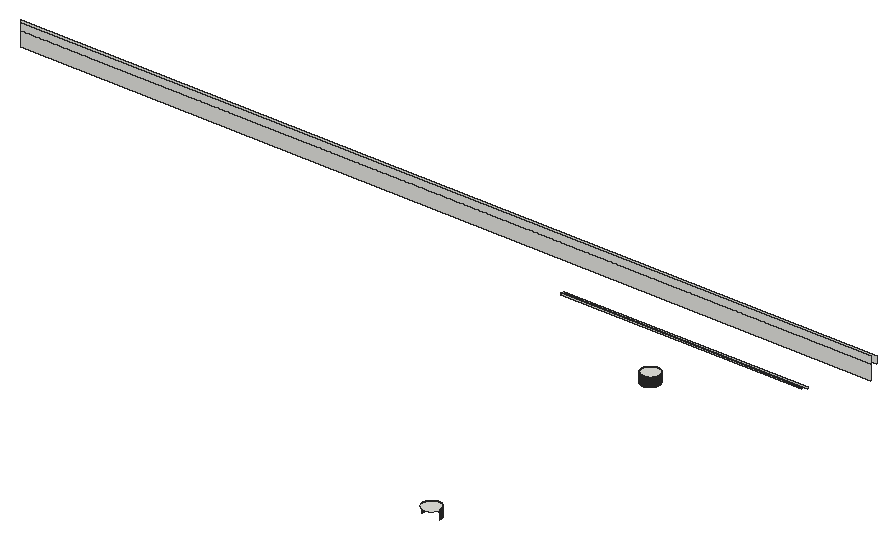
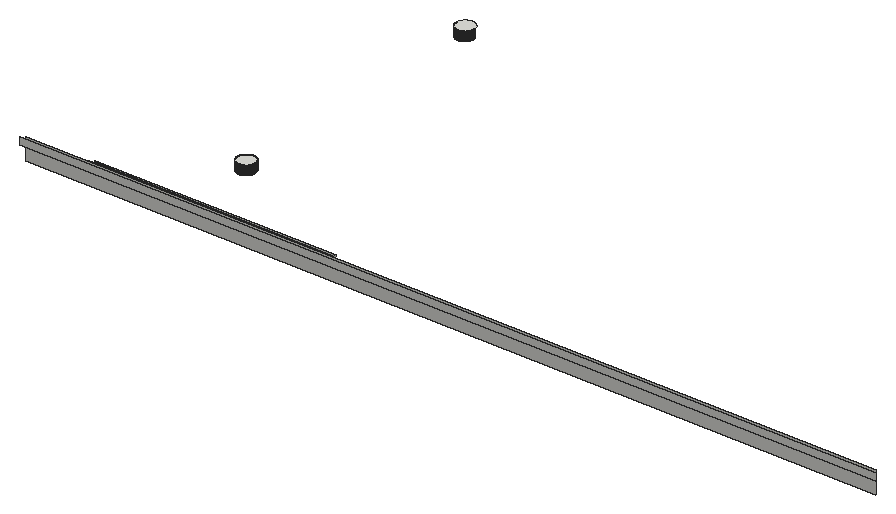
# SketchUp Ruby script. Lengths in inches.
U = 1.inch
M = Sketchup.active_model
def pt(a) = Geom::Point3d.new(a.map { |v| v * U })
def face(e, loops, mat)
  f = e.add_face(loops[0].map { |a| pt(a) })
  loops[1..].each { |l| e.add_face(l.map { |a| pt(a) }).erase! }
  f.material = f.back_material = mat if mat
  f
end
# faces: each face lists its corners as indices into pts; further lists are holes
def faces(e, pts, list, mat = nil) = list.each { |f| face(e, (f[0].is_a?(Array) ? f : [f]).map { |l| l.map { |i| pts[i] } }, mat) }
# xy, xz, yz: faces in a plane at the given z, y or x. An outline is a flat list of corners, or four numbers for a rectangle; further outlines are holes
def ring(l) = l.size == 4 ? [[l[0], l[1]], [l[2], l[1]], [l[2], l[3]], [l[0], l[3]]] : l.each_slice(2).to_a
def flat(e, list, mat, &to3) = list.each { |f| face(e, (f[0].is_a?(Array) ? f : [f]).map { |l| ring(l).map { |u, v| to3.(u, v) } }, mat) }
def xy(e, z, list, mat = nil) = flat(e, list, mat) { |x, y| [x, y, z] }
def xz(e, y, list, mat = nil) = flat(e, list, mat) { |x, z| [x, y, z] }
def yz(e, x, list, mat = nil) = flat(e, list, mat) { |y, z| [x, y, z] }
def lines(e, pts, list) = list.each { |a, b| e.add_line(pt(pts[a]), pt(pts[b])) }
# prism: a flat outline (further loops are holes) pulled along v
def prism(e, loops, v, mat = nil)
  f = face(e, loops, mat); d = Geom::Vector3d.new(v.map { |x| x * U })
  f.pushpull(f.normal.samedirection?(d) ? d.length : -d.length)
end
def box(e, o, s, mat = nil) = prism(e, [[o, [o[0] + s[0], o[1], o[2]], [o[0] + s[0], o[1] + s[1], o[2]], [o[0], o[1] + s[1], o[2]]]], [0, 0, s[2]], mat)
def at(x, y, z, deg = 0) = Geom::Transformation.translation(pt([x, y, z])) * Geom::Transformation.rotation(ORIGIN, Z_AXIS, deg.degrees)
def axes(o, x, y, z) = Geom::Transformation.new([*x, 0, *y, 0, *z, 0, *pt(o).to_a, 1])
def part(name) = M.definitions.add(name)
# library, detail: a bought-in or finely detailed component or shape, given as its bounding box
def library(name, o, s) = part(name).tap { |d| box(d.entities, o, s) }
def detail(e, o, s) = box(e.add_group.entities, o, s)
def put(e, d, t, mat = nil) = e.add_instance(d, t).tap { |i| i.material = mat if mat }
def group(e, t, mat = nil) = e.add_group.tap { |g| g.transformation = t; g.material = mat if mat }.entities
root = M.entities
xy(root,351,[[251.84,528,251.76,528.01,251.6875,528.02,251.61,528.03,251.45,528.05,251.375,528.07,251.3,528.08,251.22,528.1,251.15,528.125,251.07,528.15,251,528.17,250.92,528.2,250.71,528.29,250.64,528.33,250.57,528.36,250.43,528.44,250.37,528.48,250.3,528.53,250.24,528.57,250.17,528.62,249.93,528.82,249.88,528.88,249.77,528.99,249.62,529.17,249.57,529.24,249.53,529.3,249.48,529.37,249.44,529.43,249.36,529.57,249.33,529.64,249.29,529.71,249.23,529.85,249.2,529.93,249.17,530,249.15,530.07,249.125,530.15,249.1,530.22,249.08,530.3,249.07,530.375,249.05,530.45,249.03,530.61,249.02,530.6875,249.01,530.76,249,530.84,249,531.16,249.01,531.24,249.02,531.3125,249.03,531.39,249.05,531.55,249.07,531.625,249.08,531.7,249.1,531.78,249.125,531.85,249.15,531.93,249.17,532,249.2,532.08,249.29,532.29,249.33,532.36,249.36,532.43,249.44,532.57,249.48,532.63,249.53,532.7,249.57,532.76,249.62,532.83,249.82,533.07,249.88,533.12,249.99,533.23,250.17,533.38,250.24,533.43,250.3,533.47,250.37,533.52,250.43,533.56,250.57,533.64,250.64,533.67,250.71,533.71,250.85,533.77,250.93,533.8,251,533.83,251.07,533.85,251.15,533.875,251.22,533.9,251.3,533.92,251.375,533.93,251.45,533.95,251.61,533.97,251.6875,533.98,251.76,533.99,251.84,534,252.16,534,252.24,533.99,252.3125,533.98,252.39,533.97,252.55,533.95,252.625,533.93,252.7,533.92,252.78,533.9,252.85,533.875,252.93,533.85,253,533.83,253.08,533.8,253.29,533.71,253.36,533.67,253.43,533.64,253.57,533.56,253.63,533.52,253.7,533.47,253.76,533.43,253.83,533.38,254.07,533.18,254.12,533.12,254.23,533.01,254.38,532.83,254.43,532.76,254.47,532.7,254.52,532.63,254.56,532.57,254.64,532.43,254.67,532.36,254.71,532.29,254.77,532.15,254.8,532.07,254.83,532,254.85,531.93,254.875,531.85,254.9,531.78,254.92,531.7,254.93,531.625,254.95,531.55,254.97,531.39,254.98,531.3125,254.99,531.24,255,531.16,255,530.84,254.99,530.76,254.98,530.6875,254.97,530.61,254.95,530.45,254.93,530.375,254.92,530.3,254.9,530.22,254.875,530.15,254.85,530.07,254.83,530,254.8,529.92,254.71,529.71,254.67,529.64,254.64,529.57,254.56,529.43,254.52,529.37,254.47,529.3,254.43,529.24,254.38,529.17,254.18,528.93,254.12,528.88,254.01,528.77,253.83,528.62,253.76,528.57,253.7,528.53,253.63,528.48,253.57,528.44,253.43,528.36,253.36,528.33,253.29,528.29,253.15,528.23,253.07,528.2,253,528.17,252.93,528.15,252.85,528.125,252.78,528.1,252.7,528.08,252.625,528.07,252.55,528.05,252.39,528.03,252.3125,528.02,252.24,528.01,252.16,528],[251.84,621,251.76,621.01,251.6875,621.02,251.61,621.03,251.45,621.05,251.375,621.07,251.3,621.08,251.22,621.1,251.15,621.125,251.07,621.15,251,621.17,250.92,621.2,250.71,621.29,250.64,621.33,250.57,621.36,250.43,621.44,250.37,621.48,250.3,621.53,250.24,621.57,250.17,621.62,249.93,621.82,249.88,621.88,249.77,621.99,249.62,622.17,249.57,622.24,249.53,622.3,249.48,622.37,249.44,622.43,249.36,622.57,249.33,622.64,249.29,622.71,249.23,622.85,249.2,622.93,249.17,623,249.15,623.07,249.125,623.15,249.1,623.22,249.08,623.3,249.07,623.375,249.05,623.45,249.03,623.61,249.02,623.6875,249.01,623.76,249,623.84,249,624.16,249.01,624.24,249.02,624.3125,249.03,624.39,249.05,624.55,249.07,624.625,249.08,624.7,249.1,624.78,249.125,624.85,249.15,624.93,249.17,625,249.2,625.08,249.29,625.29,249.33,625.36,249.36,625.43,249.44,625.57,249.48,625.63,249.53,625.7,249.57,625.76,249.62,625.83,249.82,626.07,249.88,626.12,249.99,626.23,250.17,626.38,250.24,626.43,250.3,626.47,250.37,626.52,250.43,626.56,250.57,626.64,250.64,626.67,250.71,626.71,250.85,626.77,250.93,626.8,251,626.83,251.07,626.85,251.15,626.875,251.22,626.9,251.3,626.92,251.375,626.93,251.45,626.95,251.61,626.97,251.6875,626.98,251.76,626.99,251.84,627,252.16,627,252.24,626.99,252.3125,626.98,252.39,626.97,252.55,626.95,252.625,626.93,252.7,626.92,252.78,626.9,252.85,626.875,252.93,626.85,253,626.83,253.08,626.8,253.29,626.71,253.36,626.67,253.43,626.64,253.57,626.56,253.63,626.52,253.7,626.47,253.76,626.43,253.83,626.38,254.07,626.18,254.12,626.12,254.23,626.01,254.38,625.83,254.43,625.76,254.47,625.7,254.52,625.63,254.56,625.57,254.64,625.43,254.67,625.36,254.71,625.29,254.77,625.15,254.8,625.07,254.83,625,254.85,624.93,254.875,624.85,254.9,624.78,254.92,624.7,254.93,624.625,254.95,624.55,254.97,624.39,254.98,624.3125,254.99,624.24,255,624.16,255,623.84,254.99,623.76,254.98,623.6875,254.97,623.61,254.95,623.45,254.93,623.375,254.92,623.3,254.9,623.22,254.875,623.15,254.85,623.07,254.83,623,254.8,622.92,254.71,622.71,254.67,622.64,254.64,622.57,254.56,622.43,254.52,622.37,254.47,622.3,254.43,622.24,254.38,622.17,254.18,621.93,254.12,621.88,254.01,621.77,253.83,621.62,253.76,621.57,253.7,621.53,253.63,621.48,253.57,621.44,253.43,621.36,253.36,621.33,253.29,621.29,253.15,621.23,253.07,621.2,253,621.17,252.93,621.15,252.85,621.125,252.78,621.1,252.7,621.08,252.625,621.07,252.55,621.05,252.39,621.03,252.3125,621.02,252.24,621.01,252.16,621]])
xz(root,534,[[251.84,348,251.92,351],[251.92,348,252,351],[252,348,252.08,351],[252.08,348,252.16,351]])
xz(root,621,[[251.84,348,251.92,351],[251.92,348,252,351],[252,348,252.08,351],[252.08,348,252.16,351]])
xz(root,627,[[251.84,348,251.92,351],[251.92,348,252,351],[252,348,252.08,351],[252.08,348,252.16,351]])
xz(root,646,[[204,348,286,348.5]])
xz(root,647,[[204,348,287,348.5]])
xz(root,659,[[10,349.5,299,354.5],[10,354.5,299,357]])
xz(root,660,[[9,354.5,300,357]])
yz(root,204,[[646,348,647,348.5]])
yz(root,249,[[530.84,348,530.92,351],[530.92,348,531,351],[531,348,531.08,351],[531.08,348,531.16,351],[623.84,348,623.92,351],
  [623.92,348,624,351],[624,348,624.08,351],[624.08,348,624.16,351]])
yz(root,255,[[530.84,348,530.92,351],[530.92,348,531,351],[531,348,531.08,351],[531.08,348,531.16,351],[623.84,348,623.92,351],
  [623.92,348,624,351],[624,348,624.08,351],[624.08,348,624.16,351]])
p = [[249.02,530.6875,348],[249.01,530.76,348],[249.01,530.76,351],[249.02,530.6875,351],[249,530.84,348],[249,530.84,351],
  [255,530.84,348],[254.99,530.76,348],[254.99,530.76,351],[255,530.84,351],[249,531.16,348],[249.01,531.24,348],
  [249.01,531.24,351],[249,531.16,351],[249.02,531.3125,348],[249.02,531.3125,351],[254.99,531.24,348],[255,531.16,348],
  [255,531.16,351],[254.99,531.24,351],[254.98,531.3125,348],[254.98,531.3125,351],[249.03,531.39,348],[249.03,531.39,351],
  [254.97,531.39,348],[254.97,531.39,351],[249.04,531.47,348],[249.04,531.47,351],[254.96,531.47,348],[254.96,531.47,351],
  [249.05,531.55,348],[249.05,531.55,351],[249.07,531.625,348],[249.07,531.625,351],[254.95,531.55,348],[254.95,531.55,351],
  [254.93,531.625,348],[254.93,531.625,351],[249.08,531.7,348],[249.08,531.7,351],[254.92,531.7,348],[254.92,531.7,351],
  [249.1,531.78,348],[249.1,531.78,351],[254.9,531.78,348],[254.9,531.78,351],[249.125,531.85,348],[249.125,531.85,351],
  [254.875,531.85,348],[254.875,531.85,351],[249.15,531.93,348],[249.15,531.93,351],[249.17,532,348],[249.17,532,351],
  [254.83,532,348],[254.85,531.93,348],[254.85,531.93,351],[254.83,532,351],[249.2,532.08,348],[249.2,532.08,351],
  [254.8,532.07,348],[254.8,532.07,351],[249.23,532.15,348],[249.23,532.15,351],[249.26,532.22,348],[249.26,532.22,351],
  [254.74,532.22,348],[254.77,532.15,348],[254.77,532.15,351],[254.74,532.22,351],[249.29,532.29,348],[249.29,532.29,351],
  [254.71,532.29,348],[254.71,532.29,351],[249.33,532.36,348],[249.33,532.36,351],[254.67,532.36,348],[254.67,532.36,351],
  [249.36,532.43,348],[249.36,532.43,351],[249.4,532.5,348],[249.4,532.5,351],[254.64,532.43,348],[254.64,532.43,351],
  [254.6,532.5,348],[254.6,532.5,351],[249.44,532.57,348],[249.44,532.57,351],[254.56,532.57,348],[254.56,532.57,351],
  [249.48,532.63,348],[249.48,532.63,351],[249.53,532.7,348],[249.53,532.7,351],[254.52,532.63,348],[254.52,532.63,351],
  [254.47,532.7,348],[254.47,532.7,351],[249.57,532.76,348],[249.57,532.76,351],[254.43,532.76,348],[254.43,532.76,351],
  [249.62,532.83,348],[249.62,532.83,351],[249.67,532.89,348],[249.67,532.89,351],[254.33,532.89,348],[254.38,532.83,348],
  [254.38,532.83,351],[254.33,532.89,351],[249.72,532.95,348],[249.72,532.95,351],[249.77,533.01,348],[249.77,533.01,351],
  [254.23,533.01,348],[254.28,532.95,348],[254.28,532.95,351],[254.23,533.01,351],[249.82,533.07,348],[249.82,533.07,351],
  [254.18,533.06,348],[254.18,533.06,351],[249.88,533.12,348],[249.88,533.12,351],[249.94,533.18,348],[249.94,533.18,351],
  [254.12,533.12,348],[254.12,533.12,351],[254.07,533.18,348],[254.07,533.18,351],[249.99,533.23,348],[249.99,533.23,351],
  [250.05,533.28,348],[250.05,533.28,351],[253.95,533.28,348],[254.01,533.23,348],[254.01,533.23,351],[253.95,533.28,351],
  [250.11,533.33,348],[250.11,533.33,351],[250.17,533.38,348],[250.17,533.38,351],[253.83,533.38,348],[253.89,533.33,348],
  [253.89,533.33,351],[253.83,533.38,351],[250.24,533.43,348],[250.24,533.43,351],[250.3,533.47,348],[250.3,533.47,351],
  [253.7,533.47,348],[253.76,533.43,348],[253.76,533.43,351],[253.7,533.47,351],[250.37,533.52,348],[250.37,533.52,351],
  [250.43,533.56,348],[250.43,533.56,351],[253.63,533.52,348],[253.63,533.52,351],[253.57,533.56,348],[253.57,533.56,351],
  [250.5,533.6,348],[250.5,533.6,351],[250.57,533.64,348],[250.57,533.64,351],[250.64,533.67,348],[250.64,533.67,351],
  [253.43,533.64,348],[253.5,533.6,348],[253.5,533.6,351],[253.43,533.64,351],[253.36,533.67,348],[253.36,533.67,351],
  [250.71,533.71,348],[250.71,533.71,351],[250.78,533.74,348],[250.78,533.74,351],[250.85,533.77,348],[250.85,533.77,351],
  [253.15,533.77,348],[253.22,533.74,348],[253.22,533.74,351],[253.15,533.77,351],[253.29,533.71,348],[253.29,533.71,351],
  [250.93,533.8,348],[250.93,533.8,351],[251,533.83,348],[251,533.83,351],[251.07,533.85,348],[251.07,533.85,351],
  [252.93,533.85,348],[253,533.83,348],[253,533.83,351],[252.93,533.85,351],[253.08,533.8,348],[253.08,533.8,351],
  [251.15,533.875,348],[251.15,533.875,351],[251.22,533.9,348],[251.22,533.9,351],[251.3,533.92,348],[251.3,533.92,351],
  [251.375,533.93,348],[251.375,533.93,351],[251.45,533.95,348],[251.45,533.95,351],[251.53,533.96,348],[251.53,533.96,351],
  [252.55,533.95,348],[252.625,533.93,348],[252.625,533.93,351],[252.55,533.95,351],[252.47,533.96,348],[252.47,533.96,351],
  [252.7,533.92,348],[252.7,533.92,351],[252.78,533.9,348],[252.78,533.9,351],[252.85,533.875,348],[252.85,533.875,351],
  [251.61,533.97,348],[251.61,533.97,351],[251.6875,533.98,348],[251.6875,533.98,351],[251.76,533.99,348],[251.76,533.99,351],
  [251.84,534,348],[251.84,534,351],[252.24,533.99,348],[252.3125,533.98,348],[252.3125,533.98,351],[252.24,533.99,351],
  [252.16,534,348],[252.16,534,351],[252.39,533.97,348],[252.39,533.97,351],[251.61,621.03,348],[251.53,621.04,348],
  [251.53,621.04,351],[251.61,621.03,351],[251.45,621.05,348],[251.45,621.05,351],[251.6875,621.02,348],[251.6875,621.02,351],
  [251.76,621.01,348],[251.76,621.01,351],[251.84,621,348],[251.84,621,351],[252.24,621.01,348],[252.16,621,348],
  [252.16,621,351],[252.24,621.01,351],[252.3125,621.02,348],[252.3125,621.02,351],[252.39,621.03,348],[252.39,621.03,351],
  [252.47,621.04,348],[252.47,621.04,351],[252.55,621.05,348],[252.55,621.05,351],[251.07,621.15,348],[251,621.17,348],
  [251,621.17,351],[251.07,621.15,351],[251.22,621.1,348],[251.15,621.125,348],[251.15,621.125,351],[251.22,621.1,351],
  [251.3,621.08,348],[251.3,621.08,351],[251.375,621.07,348],[251.375,621.07,351],[252.625,621.07,348],[252.625,621.07,351],
  [252.7,621.08,348],[252.7,621.08,351],[252.78,621.1,348],[252.78,621.1,351],[252.85,621.125,348],[252.85,621.125,351],
  [252.93,621.15,348],[252.93,621.15,351],[253,621.17,348],[253,621.17,351],[250.85,621.23,348],[250.78,621.26,348],
  [250.78,621.26,351],[250.85,621.23,351],[250.92,621.2,348],[250.92,621.2,351],[253.07,621.2,348],[253.07,621.2,351],
  [253.15,621.23,348],[253.15,621.23,351],[253.22,621.26,348],[253.22,621.26,351],[250.71,621.29,348],[250.64,621.33,348],
  [250.64,621.33,351],[250.71,621.29,351],[250.57,621.36,348],[250.57,621.36,351],[253.29,621.29,348],[253.29,621.29,351],
  [253.36,621.33,348],[253.36,621.33,351],[253.43,621.36,348],[253.43,621.36,351],[250.5,621.4,348],[250.43,621.44,348],
  [250.43,621.44,351],[250.5,621.4,351],[250.37,621.48,348],[250.37,621.48,351],[253.5,621.4,348],[253.5,621.4,351],
  [253.57,621.44,348],[253.57,621.44,351],[253.63,621.48,348],[253.63,621.48,351],[250.3,621.53,348],[250.24,621.57,348],
  [250.24,621.57,351],[250.3,621.53,351],[253.7,621.53,348],[253.7,621.53,351],[253.76,621.57,348],[253.76,621.57,351],
  [250.17,621.62,348],[250.11,621.67,348],[250.11,621.67,351],[250.17,621.62,351],[253.83,621.62,348],[253.83,621.62,351],
  [253.89,621.67,348],[253.89,621.67,351],[250.05,621.72,348],[249.99,621.77,348],[249.99,621.77,351],[250.05,621.72,351],
  [253.95,621.72,348],[253.95,621.72,351],[254.01,621.77,348],[254.01,621.77,351],[249.93,621.82,348],[249.93,621.82,351],
  [249.88,621.88,348],[249.88,621.88,351],[254.06,621.82,348],[254.06,621.82,351],[254.12,621.88,348],[254.12,621.88,351],
  [249.82,621.94,348],[249.82,621.94,351],[249.77,621.99,348],[249.77,621.99,351],[254.18,621.93,348],[254.18,621.93,351],
  [254.23,621.99,348],[254.23,621.99,351],[249.72,622.05,348],[249.72,622.05,351],[254.28,622.05,348],[254.28,622.05,351],
  [249.67,622.11,348],[249.62,622.17,348],[249.62,622.17,351],[249.67,622.11,351],[254.33,622.11,348],[254.33,622.11,351],
  [254.38,622.17,348],[254.38,622.17,351],[249.57,622.24,348],[249.53,622.3,348],[249.53,622.3,351],[249.57,622.24,351],
  [254.43,622.24,348],[254.43,622.24,351],[254.47,622.3,348],[254.47,622.3,351],[249.48,622.37,348],[249.48,622.37,351],
  [254.52,622.37,348],[254.52,622.37,351],[249.44,622.43,348],[249.44,622.43,351],[249.4,622.5,348],[249.4,622.5,351],
  [254.56,622.43,348],[254.56,622.43,351],[254.6,622.5,348],[254.6,622.5,351],[249.36,622.57,348],[249.36,622.57,351],
  [254.64,622.57,348],[254.64,622.57,351],[249.33,622.64,348],[249.33,622.64,351],[249.29,622.71,348],[249.29,622.71,351],
  [254.67,622.64,348],[254.67,622.64,351],[254.71,622.71,348],[254.71,622.71,351],[249.26,622.78,348],[249.26,622.78,351],
  [254.74,622.78,348],[254.74,622.78,351],[249.23,622.85,348],[249.23,622.85,351],[254.77,622.85,348],[254.77,622.85,351],
  [249.2,622.93,348],[249.2,622.93,351],[249.17,623,348],[249.17,623,351],[254.8,622.92,348],[254.8,622.92,351],
  [254.83,623,348],[254.83,623,351],[249.15,623.07,348],[249.15,623.07,351],[254.85,623.07,348],[254.85,623.07,351],
  [249.125,623.15,348],[249.125,623.15,351],[249.1,623.22,348],[249.1,623.22,351],[254.875,623.15,348],[254.875,623.15,351],
  [254.9,623.22,348],[254.9,623.22,351],[249.08,623.3,348],[249.08,623.3,351],[254.92,623.3,348],[254.92,623.3,351],
  [249.07,623.375,348],[249.07,623.375,351],[254.93,623.375,348],[254.93,623.375,351],[249.05,623.45,348],[249.05,623.45,351],
  [254.95,623.45,348],[254.95,623.45,351],[249.04,623.53,348],[249.04,623.53,351],[249.03,623.61,348],[249.03,623.61,351],
  [254.96,623.53,348],[254.96,623.53,351],[254.97,623.61,348],[254.97,623.61,351],[249.02,623.6875,348],[249.02,623.6875,351],
  [254.98,623.6875,348],[254.98,623.6875,351],[249.01,623.76,348],[249.01,623.76,351],[254.99,623.76,348],[254.99,623.76,351],
  [249,623.84,348],[249,623.84,351],[255,623.84,348],[255,623.84,351],[249,624.16,348],[249.01,624.24,348],
  [249.01,624.24,351],[249,624.16,351],[249.02,624.3125,348],[249.02,624.3125,351],[254.99,624.24,348],[255,624.16,348],
  [255,624.16,351],[254.99,624.24,351],[254.98,624.3125,348],[254.98,624.3125,351],[249.03,624.39,348],[249.03,624.39,351],
  [254.97,624.39,348],[254.97,624.39,351],[249.04,624.47,348],[249.04,624.47,351],[254.96,624.47,348],[254.96,624.47,351],
  [249.05,624.55,348],[249.05,624.55,351],[249.07,624.625,348],[249.07,624.625,351],[254.95,624.55,348],[254.95,624.55,351],
  [254.93,624.625,348],[254.93,624.625,351],[249.08,624.7,348],[249.08,624.7,351],[254.92,624.7,348],[254.92,624.7,351],
  [249.1,624.78,348],[249.1,624.78,351],[254.9,624.78,348],[254.9,624.78,351],[249.125,624.85,348],[249.125,624.85,351],
  [254.875,624.85,348],[254.875,624.85,351],[249.15,624.93,348],[249.15,624.93,351],[249.17,625,348],[249.17,625,351],
  [254.83,625,348],[254.85,624.93,348],[254.85,624.93,351],[254.83,625,351],[249.2,625.08,348],[249.2,625.08,351],
  [254.8,625.07,348],[254.8,625.07,351],[249.23,625.15,348],[249.23,625.15,351],[249.26,625.22,348],[249.26,625.22,351],
  [254.74,625.22,348],[254.77,625.15,348],[254.77,625.15,351],[254.74,625.22,351],[249.29,625.29,348],[249.29,625.29,351],
  [254.71,625.29,348],[254.71,625.29,351],[249.33,625.36,348],[249.33,625.36,351],[254.67,625.36,348],[254.67,625.36,351],
  [249.36,625.43,348],[249.36,625.43,351],[249.4,625.5,348],[249.4,625.5,351],[254.64,625.43,348],[254.64,625.43,351],
  [254.6,625.5,348],[254.6,625.5,351],[249.44,625.57,348],[249.44,625.57,351],[254.56,625.57,348],[254.56,625.57,351],
  [249.48,625.63,348],[249.48,625.63,351],[249.53,625.7,348],[249.53,625.7,351],[254.52,625.63,348],[254.52,625.63,351],
  [254.47,625.7,348],[254.47,625.7,351],[249.57,625.76,348],[249.57,625.76,351],[254.43,625.76,348],[254.43,625.76,351],
  [249.62,625.83,348],[249.62,625.83,351],[249.67,625.89,348],[249.67,625.89,351],[254.33,625.89,348],[254.38,625.83,348],
  [254.38,625.83,351],[254.33,625.89,351],[249.72,625.95,348],[249.72,625.95,351],[249.77,626.01,348],[249.77,626.01,351],
  [254.23,626.01,348],[254.28,625.95,348],[254.28,625.95,351],[254.23,626.01,351],[249.82,626.07,348],[249.82,626.07,351],
  [254.18,626.06,348],[254.18,626.06,351],[249.88,626.12,348],[249.88,626.12,351],[249.94,626.18,348],[249.94,626.18,351],
  [254.12,626.12,348],[254.12,626.12,351],[254.07,626.18,348],[254.07,626.18,351],[249.99,626.23,348],[249.99,626.23,351],
  [250.05,626.28,348],[250.05,626.28,351],[253.95,626.28,348],[254.01,626.23,348],[254.01,626.23,351],[253.95,626.28,351],
  [250.11,626.33,348],[250.11,626.33,351],[250.17,626.38,348],[250.17,626.38,351],[253.83,626.38,348],[253.89,626.33,348],
  [253.89,626.33,351],[253.83,626.38,351],[250.24,626.43,348],[250.24,626.43,351],[250.3,626.47,348],[250.3,626.47,351],
  [253.7,626.47,348],[253.76,626.43,348],[253.76,626.43,351],[253.7,626.47,351],[250.37,626.52,348],[250.37,626.52,351],
  [250.43,626.56,348],[250.43,626.56,351],[253.63,626.52,348],[253.63,626.52,351],[253.57,626.56,348],[253.57,626.56,351],
  [250.5,626.6,348],[250.5,626.6,351],[250.57,626.64,348],[250.57,626.64,351],[250.64,626.67,348],[250.64,626.67,351],
  [253.43,626.64,348],[253.5,626.6,348],[253.5,626.6,351],[253.43,626.64,351],[253.36,626.67,348],[253.36,626.67,351],
  [250.71,626.71,348],[250.71,626.71,351],[250.78,626.74,348],[250.78,626.74,351],[250.85,626.77,348],[250.85,626.77,351],
  [253.15,626.77,348],[253.22,626.74,348],[253.22,626.74,351],[253.15,626.77,351],[253.29,626.71,348],[253.29,626.71,351],
  [250.93,626.8,348],[250.93,626.8,351],[251,626.83,348],[251,626.83,351],[251.07,626.85,348],[251.07,626.85,351],
  [252.93,626.85,348],[253,626.83,348],[253,626.83,351],[252.93,626.85,351],[253.08,626.8,348],[253.08,626.8,351],
  [251.15,626.875,348],[251.15,626.875,351],[251.22,626.9,348],[251.22,626.9,351],[251.3,626.92,348],[251.3,626.92,351],
  [251.375,626.93,348],[251.375,626.93,351],[251.45,626.95,348],[251.45,626.95,351],[251.53,626.96,348],[251.53,626.96,351],
  [252.55,626.95,348],[252.625,626.93,348],[252.625,626.93,351],[252.55,626.95,351],[252.47,626.96,348],[252.47,626.96,351],
  [252.7,626.92,348],[252.7,626.92,351],[252.78,626.9,348],[252.78,626.9,351],[252.85,626.875,348],[252.85,626.875,351],
  [251.61,626.97,348],[251.61,626.97,351],[251.6875,626.98,348],[251.6875,626.98,351],[251.76,626.99,348],[251.76,626.99,351],
  [251.84,627,348],[251.84,627,351],[252.24,626.99,348],[252.3125,626.98,348],[252.3125,626.98,351],[252.24,626.99,351],
  [252.16,627,348],[252.16,627,351],[252.39,626.97,348],[252.39,626.97,351]]
faces(root,p,[[0,1,2,3],[1,4,5,2],[6,7,8,9],[10,11,12,13],[11,14,15,12],[16,17,18,19],[20,16,19,21],[14,22,23,15],
  [24,20,21,25],[22,26,27,23],[28,24,25,29],[26,30,31,27],[30,32,33,31],[34,28,29,35],[36,34,35,37],[32,38,39,33],
  [40,36,37,41],[38,42,43,39],[44,40,41,45],[42,46,47,43],[48,44,45,49],[46,50,51,47],[50,52,53,51],[54,55,56,57],
  [55,48,49,56],[52,58,59,53],[60,54,57,61],[58,62,63,59],[62,64,65,63],[66,67,68,69],[67,60,61,68],[64,70,71,65],
  [72,66,69,73],[70,74,75,71],[76,72,73,77],[74,78,79,75],[78,80,81,79],[82,76,77,83],[84,82,83,85],[80,86,87,81],
  [88,84,85,89],[86,90,91,87],[90,92,93,91],[94,88,89,95],[96,94,95,97],[92,98,99,93],[100,96,97,101],[98,102,103,99],
  [102,104,105,103],[106,107,108,109],[107,100,101,108],[104,110,111,105],[110,112,113,111],[114,115,116,117],[115,106,109,116],[112,118,119,113],
  [120,114,117,121],[118,122,123,119],[122,124,125,123],[126,120,121,127],[128,126,127,129],[124,130,131,125],[130,132,133,131],[134,135,136,137],
  [135,128,129,136],[132,138,139,133],[138,140,141,139],[142,143,144,145],[143,134,137,144],[140,146,147,141],[146,148,149,147],[150,151,152,153],
  [151,142,145,152],[148,154,155,149],[154,156,157,155],[158,150,153,159],[160,158,159,161],[156,162,163,157],[162,164,165,163],[164,166,167,165],
  [168,169,170,171],[172,168,171,173],[169,160,161,170],[166,174,175,167],[174,176,177,175],[176,178,179,177],[180,181,182,183],[181,184,185,182],
  [184,172,173,185],[178,186,187,179],[186,188,189,187],[188,190,191,189],[192,193,194,195],[193,196,197,194],[196,180,183,197],[190,198,199,191],
  [198,200,201,199],[200,202,203,201],[202,204,205,203],[204,206,207,205],[206,208,209,207],[210,211,212,213],[214,210,213,215],[211,216,217,212],
  [216,218,219,217],[218,220,221,219],[220,192,195,221],[208,222,223,209],[222,224,225,223],[224,226,227,225],[226,228,229,227],[230,231,232,233],
  [234,230,233,235],[231,236,237,232],[236,214,215,237],[238,239,240,241],[239,242,243,240],[244,238,241,245],[246,244,245,247],[248,246,247,249],
  [250,251,252,253],[254,250,253,255],[256,254,255,257],[258,256,257,259],[260,258,259,261],[262,263,264,265],[266,267,268,269],[267,262,265,268],
  [270,266,269,271],[272,270,271,273],[242,272,273,243],[274,260,261,275],[276,274,275,277],[278,276,277,279],[280,278,279,281],[282,280,281,283],
  [284,282,283,285],[286,287,288,289],[263,290,291,264],[290,286,289,291],[292,284,285,293],[294,292,293,295],[296,294,295,297],[298,299,300,301],
  [299,302,303,300],[287,298,301,288],[304,296,297,305],[306,304,305,307],[308,306,307,309],[310,311,312,313],[311,314,315,312],[302,310,313,303],
  [316,308,309,317],[318,316,317,319],[320,318,319,321],[322,323,324,325],[314,322,325,315],[326,320,321,327],[328,326,327,329],[330,331,332,333],
  [323,330,333,324],[334,328,329,335],[336,334,335,337],[338,339,340,341],[331,338,341,332],[342,336,337,343],[344,342,343,345],[339,346,347,340],
  [346,348,349,347],[350,344,345,351],[352,350,351,353],[348,354,355,349],[354,356,357,355],[358,352,353,359],[360,358,359,361],[356,362,363,357],
  [364,360,361,365],[366,367,368,369],[362,366,369,363],[370,364,365,371],[372,370,371,373],[374,375,376,377],[367,374,377,368],[378,372,373,379],
  [380,378,379,381],[375,382,383,376],[384,380,381,385],[382,386,387,383],[386,388,389,387],[390,384,385,391],[392,390,391,393],[388,394,395,389],
  [396,392,393,397],[394,398,399,395],[398,400,401,399],[402,396,397,403],[404,402,403,405],[400,406,407,401],[408,404,405,409],[406,410,411,407],
  [412,408,409,413],[410,414,415,411],[414,416,417,415],[418,412,413,419],[420,418,419,421],[416,422,423,417],[424,420,421,425],[422,426,427,423],
  [426,428,429,427],[430,424,425,431],[432,430,431,433],[428,434,435,429],[436,432,433,437],[434,438,439,435],[440,436,437,441],[438,442,443,439],
  [444,440,441,445],[442,446,447,443],[446,448,449,447],[450,444,445,451],[452,450,451,453],[448,454,455,449],[456,452,453,457],[454,458,459,455],
  [460,456,457,461],[458,462,463,459],[464,460,461,465],[466,467,468,469],[467,470,471,468],[472,473,474,475],[476,472,475,477],[470,478,479,471],
  [480,476,477,481],[478,482,483,479],[484,480,481,485],[482,486,487,483],[486,488,489,487],[490,484,485,491],[492,490,491,493],[488,494,495,489],
  [496,492,493,497],[494,498,499,495],[500,496,497,501],[498,502,503,499],[504,500,501,505],[502,506,507,503],[506,508,509,507],[510,511,512,513],
  [511,504,505,512],[508,514,515,509],[516,510,513,517],[514,518,519,515],[518,520,521,519],[522,523,524,525],[523,516,517,524],[520,526,527,521],
  [528,522,525,529],[526,530,531,527],[532,528,529,533],[530,534,535,531],[534,536,537,535],[538,532,533,539],[540,538,539,541],[536,542,543,537],
  [544,540,541,545],[542,546,547,543],[546,548,549,547],[550,544,545,551],[552,550,551,553],[548,554,555,549],[556,552,553,557],[554,558,559,555],
  [558,560,561,559],[562,563,564,565],[563,556,557,564],[560,566,567,561],[566,568,569,567],[570,571,572,573],[571,562,565,572],[568,574,575,569],
  [576,570,573,577],[574,578,579,575],[578,580,581,579],[582,576,577,583],[584,582,583,585],[580,586,587,581],[586,588,589,587],[590,591,592,593],
  [591,584,585,592],[588,594,595,589],[594,596,597,595],[598,599,600,601],[599,590,593,600],[596,602,603,597],[602,604,605,603],[606,607,608,609],
  [607,598,601,608],[604,610,611,605],[610,612,613,611],[614,606,609,615],[616,614,615,617],[612,618,619,613],[618,620,621,619],[620,622,623,621],
  [624,625,626,627],[628,624,627,629],[625,616,617,626],[622,630,631,623],[630,632,633,631],[632,634,635,633],[636,637,638,639],[637,640,641,638],
  [640,628,629,641],[634,642,643,635],[642,644,645,643],[644,646,647,645],[648,649,650,651],[649,652,653,650],[652,636,639,653],[646,654,655,647],
  [654,656,657,655],[656,658,659,657],[658,660,661,659],[660,662,663,661],[662,664,665,663],[666,667,668,669],[670,666,669,671],[667,672,673,668],
  [672,674,675,673],[674,676,677,675],[676,648,651,677],[664,678,679,665],[678,680,681,679],[680,682,683,681],[682,684,685,683],[686,687,688,689],
  [690,686,689,691],[687,692,693,688],[692,670,671,693]])
